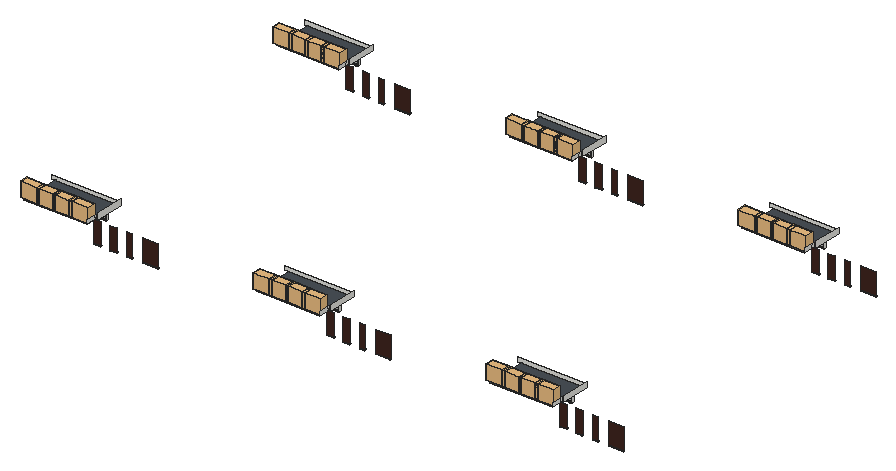
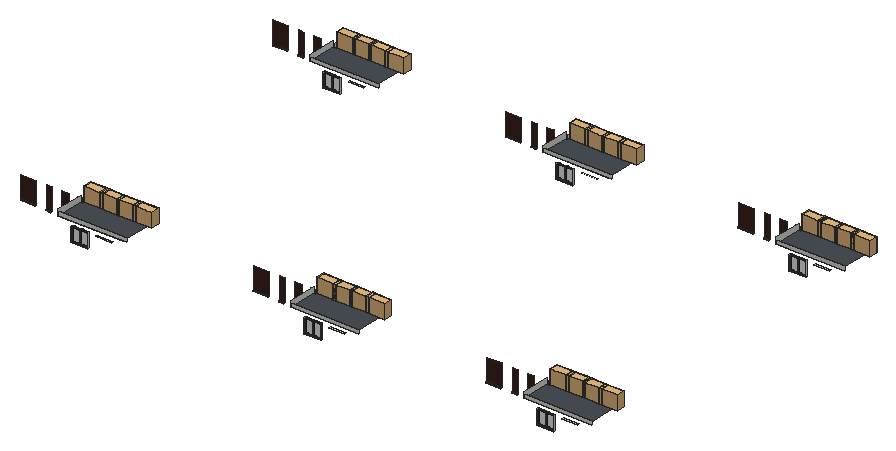
# SketchUp Ruby script. Lengths in inches.
U = 1.inch
M = Sketchup.active_model
def pt(a) = Geom::Point3d.new(a.map { |v| v * U })
def face(e, loops, mat)
  f = e.add_face(loops[0].map { |a| pt(a) })
  loops[1..].each { |l| e.add_face(l.map { |a| pt(a) }).erase! }
  f.material = f.back_material = mat if mat
  f
end
# faces: each face lists its corners as indices into pts; further lists are holes
def faces(e, pts, list, mat = nil) = list.each { |f| face(e, (f[0].is_a?(Array) ? f : [f]).map { |l| l.map { |i| pts[i] } }, mat) }
# xy, xz, yz: faces in a plane at the given z, y or x. An outline is a flat list of corners, or four numbers for a rectangle; further outlines are holes
def ring(l) = l.size == 4 ? [[l[0], l[1]], [l[2], l[1]], [l[2], l[3]], [l[0], l[3]]] : l.each_slice(2).to_a
def flat(e, list, mat, &to3) = list.each { |f| face(e, (f[0].is_a?(Array) ? f : [f]).map { |l| ring(l).map { |u, v| to3.(u, v) } }, mat) }
def xy(e, z, list, mat = nil) = flat(e, list, mat) { |x, y| [x, y, z] }
def xz(e, y, list, mat = nil) = flat(e, list, mat) { |x, z| [x, y, z] }
def yz(e, x, list, mat = nil) = flat(e, list, mat) { |y, z| [x, y, z] }
def lines(e, pts, list) = list.each { |a, b| e.add_line(pt(pts[a]), pt(pts[b])) }
# prism: a flat outline (further loops are holes) pulled along v
def prism(e, loops, v, mat = nil)
  f = face(e, loops, mat); d = Geom::Vector3d.new(v.map { |x| x * U })
  f.pushpull(f.normal.samedirection?(d) ? d.length : -d.length)
end
def box(e, o, s, mat = nil) = prism(e, [[o, [o[0] + s[0], o[1], o[2]], [o[0] + s[0], o[1] + s[1], o[2]], [o[0], o[1] + s[1], o[2]]]], [0, 0, s[2]], mat)
def at(x, y, z, deg = 0) = Geom::Transformation.translation(pt([x, y, z])) * Geom::Transformation.rotation(ORIGIN, Z_AXIS, deg.degrees)
def axes(o, x, y, z) = Geom::Transformation.new([*x, 0, *y, 0, *z, 0, *pt(o).to_a, 1])
def part(name) = M.definitions.add(name)
# library, detail: a bought-in or finely detailed component or shape, given as its bounding box
def library(name, o, s) = part(name).tap { |d| box(d.entities, o, s) }
def detail(e, o, s) = box(e.add_group.entities, o, s)
def put(e, d, t, mat = nil) = e.add_instance(d, t).tap { |i| i.material = mat if mat }
def group(e, t, mat = nil) = e.add_group.tap { |g| g.transformation = t; g.material = mat if mat }.entities
root = M.entities
M.materials.add("Glass_Tinted_Gray").color = [0, 0, 0]
M.materials["Glass_Tinted_Gray"].alpha = 0.125
M.materials.add("[0043_SaddleBrown]").color = [63, 38, 31]
M.materials.add("[0135_DarkGray]").color = [81, 81, 81]
M.materials.add("[Formica Blue]").color = [73, 80, 86]
M.materials.add("[Mirror 02]").color = [229, 229, 229]
M.materials.add("[Terrazzo Light Blue]").color = [196, 214, 227]
c1 = part("PENTEK_RP Fineline 50S_Sliding_DoorCase_E1")
box(c1.entities,[0,0,0],[1.51,3.66,99.27],"[0135_DarkGray]")
c2 = part("PENTEK_RP Fineline 50S_SlidingDooe_Case_E2")
box(c2.entities,[0,0,0],[96.25,3.66,1.51],"[0135_DarkGray]")
c3 = part("pentek_RP Fineline 50S_SlidingDoor_Case")
put(c3.entities,c1,at(97.76,0,0))
put(c3.entities,c2,at(1.51,0,0))
put(c3.entities,c1,at(0,0,0))
put(c3.entities,c2,at(1.51,0,97.76))
c4 = part("PENTEK_RP Fineline 50S_SlidingDoor_GlazingBead_2")
box(c4.entities,[0,0,0],[0.56,0.59,94.39],"[0135_DarkGray]")
c5 = part("PENTEK_RP Fineline 50S_SlidingDoor_Glass")
box(c5.entities,[0,0,0],[46.58,0.16,94.39],"Glass_Tinted_Gray")
c6 = part("PENTEK_RP Fineline 50S_SlidingDoor_GlazingBead")
box(c6.entities,[0,0,0],[45.47,0.59,0.56],"[0135_DarkGray]")
c7 = part("PENTEK_RP Fineline 50S_SlidingDoor_Leaf_E1")
xy(c7.entities,0,[[0,0,0.93,1.97],[0.93,1.57,1.49,1.97]],"[0135_DarkGray]")
xy(c7.entities,96.25,[[0,0,0.93,0,0.93,1.57,1.49,1.57,1.49,1.97,0,1.97]],"[0135_DarkGray]")
xz(c7.entities,0,[[0,0,0.93,96.25]],"[0135_DarkGray]")
xz(c7.entities,1.57,[[0.93,0,1.49,95.32],[0.93,95.32,1.49,96.25]],"[0135_DarkGray]")
xz(c7.entities,1.97,[[0,0,1.49,96.25]],"[0135_DarkGray]")
yz(c7.entities,0,[[0,0,1.97,96.25]],"[0135_DarkGray]")
yz(c7.entities,0.93,[[0,0,1.57,0.93],[0,0.93,1.57,95.32],[0,95.32,1.57,96.25]],"[0135_DarkGray]")
yz(c7.entities,1.49,[[1.57,0,1.97,95.32],[1.57,95.32,1.97,96.25]],"[0135_DarkGray]")
c8 = part("PENTEK_RP Fineline 50S_SlidingDoor_Leaf_E2")
xy(c8.entities,0,[[0,0,0,1.57,0.56,1.57,0.56,1.97,46.02,1.97,46.02,1.57,46.58,1.57,46.58,0]],"[0135_DarkGray]")
xy(c8.entities,0.93,[[0,0,46.58,1.57]],"[0135_DarkGray]")
xy(c8.entities,1.49,[[0.56,1.57,46.02,1.97]],"[0135_DarkGray]")
xz(c8.entities,0,[[0,0,46.58,0.93]],"[0135_DarkGray]")
xz(c8.entities,1.57,[[0,0,0.56,0.93],[46.02,0,46.58,0.93],[0.56,0.93,46.02,1.49]],"[0135_DarkGray]")
xz(c8.entities,1.97,[[0.56,0,46.02,1.49]],"[0135_DarkGray]")
yz(c8.entities,0,[[0,0,1.57,0.93]],"[0135_DarkGray]")
yz(c8.entities,0.56,[[1.57,0,1.97,0.93],[1.57,0.93,1.97,1.49]],"[0135_DarkGray]")
yz(c8.entities,46.02,[[1.57,0,1.97,0.93],[1.57,0.93,1.97,1.49]],"[0135_DarkGray]")
yz(c8.entities,46.58,[[0,0,1.57,0.93]],"[0135_DarkGray]")
c9 = part("PENTEK_RP Fineline S_SlidingDoor_Leaf1")
put(c9.entities,c4,at(0.93,0,0.93))
put(c9.entities,c4,at(46.96,0,0.93))
put(c9.entities,c5,at(1.49,1.42,0.93))
put(c9.entities,c6,at(1.49,0,0.93))
put(c9.entities,c5,at(1.49,0.59,0.93),"[Terrazzo Light Blue]")
put(c9.entities,c7,at(0,0,0))
put(c9.entities,c7,axes([48.44,0,0],[-1,0,0],[0,1,0],[0,0,1]))
put(c9.entities,c8,axes([0.93,0,96.25],[1,0,0],[0,1,0],[0,0,-1]))
put(c9.entities,c8,at(0.93,0,0))
put(c9.entities,c6,at(1.49,0,94.77))
c10 = part("PENTEK_RP Fineline 50S_SlidingDoor_Leaf2")
put(c10.entities,c5,at(1.49,1.42,0.93))
put(c10.entities,c6,at(1.49,0,94.77))
put(c10.entities,c4,at(46.96,0,0.93))
put(c10.entities,c5,at(1.49,0.59,0.93),"[Mirror 02]")
put(c10.entities,c4,at(0.93,0,0.93))
put(c10.entities,c7,at(0,0,0))
put(c10.entities,c7,axes([48.44,0,0],[-1,0,0],[0,1,0],[0,0,1]))
put(c10.entities,c6,at(1.49,0,0.93))
put(c10.entities,c8,axes([0.93,0,96.25],[1,0,0],[0,1,0],[0,0,-1]))
put(c10.entities,c8,at(0.93,0,0))
c11 = part("PENTEK - Slimmest Steel Sliding Door / Window\#1")
put(c11.entities,c3,at(0,-1.88,-0.09))
put(c11.entities,c9,at(1.51,-2.27,1.42))
put(c11.entities,c10,at(49.32,-0.3,1.42))
c12 = library("Group13",[-203.48,36.63,0],[29.68,67.31,50.64])
xy(root,173.82,[[451.01,438.72,467.3,441.04],[1175.45,438.72,1191.74,441.04],[1899.89,438.72,1916.17,441.04],[451.01,1419.07,467.3,1421.39],[1175.45,1419.07,1191.74,1421.39],
  [1899.89,1419.07,1916.17,1421.39]])
xy(root,173.87,[[419.76,438.72,419.76,441.04,399.16,441.04,399.16,438.73],[1144.2,438.72,1144.2,441.04,1123.6,441.04,1123.6,438.73],[1868.64,438.72,1868.64,441.04,1848.04,441.04,1848.04,438.73],[419.76,1419.07,419.76,1421.39,399.16,1421.39,399.16,1419.08],[1144.2,1419.07,1144.2,1421.39,1123.6,1421.39,1123.6,1419.08],
  [1868.64,1419.07,1868.64,1421.39,1848.04,1421.39,1848.04,1419.08]])
xy(root,174.69,[[348.1875,438.72,370.54,441.04],[1072.625,438.72,1094.98,441.04],[1797.0625,438.72,1819.41,441.04],[348.1875,1419.07,370.54,1419.08,370.54,1421.39,348.1875,1421.39],[1072.625,1419.07,1094.98,1419.08,1094.98,1421.39,1072.625,1421.39],
  [1797.0625,1419.07,1819.41,1419.08,1819.41,1421.39,1797.0625,1421.39]])
xy(root,174.81,[[500.42,438.73,547.05,441.04],[1224.86,438.73,1271.49,441.04],[1949.3,438.73,1995.93,441.04],[500.42,1419.08,547.05,1421.39],[1224.86,1419.08,1271.49,1421.39],
  [1949.3,1419.08,1995.93,1421.39]])
xy(root,175.12,[[419.76,438.72,399.16,438.73,399.16,441.04,419.76,441.04],[1144.2,438.72,1123.6,438.73,1123.6,441.04,1144.2,441.04],[1868.64,438.72,1848.04,438.73,1848.04,441.04,1868.64,441.04],[419.76,1419.07,399.16,1419.08,399.16,1421.39,419.76,1421.39],[1144.2,1419.07,1123.6,1419.08,1123.6,1421.39,1144.2,1421.39],
  [1868.64,1419.07,1848.04,1419.08,1848.04,1421.39,1868.64,1421.39]])
xy(root,175.93,[[451.01,438.72,467.3,441.04],[1175.45,438.72,1191.74,441.04],[1899.89,438.72,1916.17,441.04],[451.01,1419.07,467.3,1421.39],[1175.45,1419.07,1191.74,1421.39],
  [1899.89,1419.07,1916.17,1421.39]])
xy(root,176.39,[[348.1875,438.72,370.54,441.04],[1072.625,438.72,1094.98,441.04],[1797.0625,438.72,1819.41,441.04],[348.1875,1419.07,370.54,1421.39],[1072.625,1419.07,1094.98,1421.39],
  [1797.0625,1419.07,1819.41,1421.39]])
xy(root,177.22,[[500.42,438.73,547.05,441.04],[1224.86,438.73,1271.49,441.04],[1949.3,438.73,1995.93,441.04],[500.42,1419.08,547.05,1421.39],[1224.86,1419.08,1271.49,1421.39],
  [1949.3,1419.08,1995.93,1421.39]])
xy(root,183.6875,[[258.09,535.375,309.84,540.48],[982.53,535.375,1034.28,540.48],[1706.96,535.375,1758.71,540.48],[258.09,1515.73,309.84,1520.83],[982.53,1515.73,1034.28,1520.83],
  [1706.96,1515.73,1758.71,1520.83]])
xy(root,227.875,[[183.3,535.375,231.3,540.48],[258.09,535.375,309.84,540.48],[907.74,535.375,955.74,540.48],[982.53,535.375,1034.28,540.48],[1632.17,535.375,1680.17,540.48],
  [1706.96,535.375,1758.71,540.48],[183.3,1515.73,231.3,1520.83],[258.09,1515.73,309.84,1520.83],[907.74,1515.73,955.74,1520.83],[982.53,1515.73,1034.28,1520.83],
  [1632.17,1515.73,1680.17,1520.83],[1706.96,1515.73,1758.71,1520.83]])
xy(root,240.625,[[[153.26,412.04,153.26,535.375,353.97,535.375,353.97,447.84,348.1875,447.84,348.1875,412.04],[154.69,414.01,158.32,418.7],[160.01,414.01,163.63,418.7],[165.19,414.01,168.82,418.7],[170.38,414.01,174.01,418.7],[181.38,414.01,185.01,418.7],[186.88,414.01,190.51,418.7],[192.38,414.01,196.01,418.7],[197.88,414.01,201.51,418.7],[203.38,414.01,207.01,418.7],[175.88,414.01,179.51,418.7]],[[877.69,412.04,877.69,535.375,1078.41,535.375,1078.41,447.84,1072.625,447.84,1072.625,412.04],[879.13,414.01,882.76,418.7],[884.44,414.01,888.07,418.7],[889.63,414.01,893.26,418.7],[894.82,414.01,898.44,418.7],[900.32,414.01,903.94,418.7],[905.82,414.01,909.44,418.7],[911.32,414.01,914.94,418.7],[916.82,414.01,920.44,418.7],[922.32,414.01,925.94,418.7],[927.82,414.01,931.44,418.7]],[[1602.13,412.04,1602.13,535.375,1802.84,535.375,1802.84,447.84,1797.0625,447.84,1797.0625,412.04],[1603.57,414.01,1607.19,418.7],[1608.88,414.01,1612.51,418.7],[1614.07,414.01,1617.69,418.7],[1619.26,414.01,1622.88,418.7],[1630.26,414.01,1633.88,418.7],[1635.76,414.01,1639.38,418.7],[1641.26,414.01,1644.88,418.7],[1646.76,414.01,1650.38,418.7],[1652.26,414.01,1655.88,418.7],[1624.76,414.01,1628.38,418.7]],[[153.26,1392.39,153.26,1515.73,353.97,1515.73,353.97,1428.19,348.1875,1428.19,348.1875,1392.39],[154.69,1394.36,158.32,1399.05],[160.01,1394.36,163.63,1399.05],[165.19,1394.36,168.82,1399.05],[170.38,1394.36,174.01,1399.05],[181.38,1394.36,185.01,1399.05],[186.88,1394.36,190.51,1399.05],[192.38,1394.36,196.01,1399.05],[197.88,1394.36,201.51,1399.05],[203.38,1394.36,207.01,1399.05],[175.88,1394.36,179.51,1399.05]],[[877.69,1392.39,877.69,1515.73,1078.41,1515.73,1078.41,1428.19,1072.625,1428.19,1072.625,1392.39],[879.13,1394.36,882.76,1399.05],[884.44,1394.36,888.07,1399.05],[889.63,1394.36,893.26,1399.05],[894.82,1394.36,898.44,1399.05],[900.32,1394.36,903.94,1399.05],[905.82,1394.36,909.44,1399.05],[911.32,1394.36,914.94,1399.05],[916.82,1394.36,920.44,1399.05],[922.32,1394.36,925.94,1399.05],[927.82,1394.36,931.44,1399.05]],
  [[1602.13,1392.39,1602.13,1515.73,1802.84,1515.73,1802.84,1428.19,1797.0625,1428.19,1797.0625,1392.39],[1603.57,1394.36,1607.19,1399.05],[1608.88,1394.36,1612.51,1399.05],[1614.07,1394.36,1617.69,1399.05],[1619.26,1394.36,1622.88,1399.05],[1630.26,1394.36,1633.88,1399.05],[1635.76,1394.36,1639.38,1399.05],[1641.26,1394.36,1644.88,1399.05],[1646.76,1394.36,1650.38,1399.05],[1652.26,1394.36,1655.88,1399.05],[1624.76,1394.36,1628.38,1399.05]]],"[Formica Blue]")
xz(root,438.72,[[451.01,175.93,467.3,243.96],[1175.45,175.93,1191.74,243.96],[1899.89,175.93,1916.17,243.96],[348.1875,176.39,370.54,243.96],[1072.625,176.39,1094.98,243.96],
  [1797.0625,176.39,1819.41,243.96]],"[0043_SaddleBrown]")
xz(root,438.73,[[500.42,177.22,547.05,243.96],[1224.86,177.22,1271.49,243.96],[1949.3,177.22,1995.93,243.96]],"[0043_SaddleBrown]")
xz(root,441.04,[[451.01,173.82,467.3,175.93],[1175.45,173.82,1191.74,175.93],[1899.89,173.82,1916.17,175.93],[399.16,173.87,419.76,175.12],[1123.6,173.87,1144.2,175.12],
  [1848.04,173.87,1868.64,175.12],[348.1875,174.69,370.54,176.39],[1072.625,174.69,1094.98,176.39],[1797.0625,174.69,1819.41,176.39],[500.42,174.81,547.05,177.22],
  [1224.86,174.81,1271.49,177.22],[1949.3,174.81,1995.93,177.22]],"[0043_SaddleBrown]")
xz(root,447.84,[[348.1875,240.625,353.97,252.25],[1072.625,240.625,1078.41,252.25],[1797.0625,240.625,1802.84,252.25]])
xz(root,535.375,[[141.63,240.625,353.97,252.25],[866.07,240.625,1078.41,252.25],[1590.51,240.625,1802.84,252.25]])
xz(root,1419.07,[[451.01,175.93,467.3,243.96],[1175.45,175.93,1191.74,243.96],[1899.89,175.93,1916.17,243.96],[348.1875,176.39,370.54,243.96],[1072.625,176.39,1094.98,243.96],
  [1797.0625,176.39,1819.41,243.96]],"[0043_SaddleBrown]")
xz(root,1419.08,[[500.42,177.22,547.05,243.96],[1224.86,177.22,1271.49,243.96],[1949.3,177.22,1995.93,243.96]],"[0043_SaddleBrown]")
xz(root,1421.39,[[451.01,173.82,467.3,175.93],[1175.45,173.82,1191.74,175.93],[1899.89,173.82,1916.17,175.93],[399.16,173.87,419.76,175.12],[1123.6,173.87,1144.2,175.12],
  [1848.04,173.87,1868.64,175.12],[348.1875,174.69,370.54,176.39],[1072.625,174.69,1094.98,176.39],[1797.0625,174.69,1819.41,176.39],[500.42,174.81,547.05,177.22],
  [1224.86,174.81,1271.49,177.22],[1949.3,174.81,1995.93,177.22]],"[0043_SaddleBrown]")
xz(root,1428.19,[[348.1875,240.625,353.97,252.25],[1072.625,240.625,1078.41,252.25],[1797.0625,240.625,1802.84,252.25]])
xz(root,1515.73,[[141.63,240.625,353.97,252.25],[866.07,240.625,1078.41,252.25],[1590.51,240.625,1802.84,252.25]])
yz(root,258.09,[[535.375,183.6875,540.48,227.875],[1515.73,183.6875,1520.83,227.875]])
yz(root,309.84,[[535.375,183.6875,540.48,227.875],[1515.73,183.6875,1520.83,227.875]])
yz(root,348.1875,[[412.04,240.625,438.72,240.625,438.72,243.96,441.04,243.96,441.04,246.4375,438.72,246.4375,438.72,252.25,412.04,252.25],[438.72,240.625,438.72,243.96,441.04,243.96,441.04,246.4375,438.72,246.4375,438.72,252.25,447.84,252.25,447.84,240.625],[1392.39,240.625,1419.07,240.625,1419.07,243.96,1421.39,243.96,1421.39,246.4375,1419.07,246.4375,1419.07,252.25,1392.39,252.25],[1419.07,240.625,1419.07,243.96,1421.39,243.96,1421.39,246.4375,1419.07,246.4375,1419.07,252.25,1428.19,252.25,1428.19,240.625]])
yz(root,353.97,[[447.84,240.625,535.375,258.25],[1428.19,240.625,1515.73,258.25]])
yz(root,982.53,[[535.375,183.6875,540.48,227.875],[1515.73,183.6875,1520.83,227.875]])
yz(root,1034.28,[[535.375,183.6875,540.48,227.875],[1515.73,183.6875,1520.83,227.875]])
yz(root,1072.625,[[412.04,240.625,438.72,240.625,438.72,243.96,441.04,243.96,441.04,246.4375,438.72,246.4375,438.72,252.25,412.04,252.25],[438.72,240.625,438.72,243.96,441.04,243.96,441.04,246.4375,438.72,246.4375,438.72,252.25,447.84,252.25,447.84,240.625],[1392.39,240.625,1419.07,240.625,1419.07,243.96,1421.39,243.96,1421.39,246.4375,1419.07,246.4375,1419.07,252.25,1392.39,252.25],[1419.07,240.625,1419.07,243.96,1421.39,243.96,1421.39,246.4375,1419.07,246.4375,1419.07,252.25,1428.19,252.25,1428.19,240.625]])
yz(root,1078.41,[[447.84,240.625,535.375,258.25],[1428.19,240.625,1515.73,258.25]])
yz(root,1706.96,[[535.375,183.6875,540.48,227.875],[1515.73,183.6875,1520.83,227.875]])
yz(root,1758.71,[[535.375,183.6875,540.48,227.875],[1515.73,183.6875,1520.83,227.875]])
yz(root,1797.0625,[[412.04,240.625,438.72,240.625,438.72,243.96,441.04,243.96,441.04,246.4375,438.72,246.4375,438.72,252.25,412.04,252.25],[438.72,240.625,438.72,243.96,441.04,243.96,441.04,246.4375,438.72,246.4375,438.72,252.25,447.84,252.25,447.84,240.625],[1392.39,240.625,1419.07,240.625,1419.07,243.96,1421.39,243.96,1421.39,246.4375,1419.07,246.4375,1419.07,252.25,1392.39,252.25],[1419.07,240.625,1419.07,243.96,1421.39,243.96,1421.39,246.4375,1419.07,246.4375,1419.07,252.25,1428.19,252.25,1428.19,240.625]])
yz(root,1802.84,[[447.84,240.625,535.375,258.25],[1428.19,240.625,1515.73,258.25]])
p = [[399.16,438.72,243.96],[399.16,438.73,175.12],[419.76,438.72,175.12],[419.76,438.72,243.96],[1123.6,438.72,243.96],[1123.6,438.73,175.12],
  [1144.2,438.72,175.12],[1144.2,438.72,243.96],[1848.04,438.72,243.96],[1848.04,438.73,175.12],[1868.64,438.72,175.12],[1868.64,438.72,243.96],
  [399.16,1419.07,243.96],[399.16,1419.08,175.12],[419.76,1419.07,175.12],[419.76,1419.07,243.96],[1123.6,1419.07,243.96],[1123.6,1419.08,175.12],
  [1144.2,1419.07,175.12],[1144.2,1419.07,243.96],[1848.04,1419.07,243.96],[1848.04,1419.08,175.12],[1868.64,1419.07,175.12],[1868.64,1419.07,243.96]]
faces(root,p,[[0,1,2,3],[4,5,6,7],[8,9,10,11],[12,13,14,15],[16,17,18,19],[20,21,22,23]],"[0043_SaddleBrown]")
put(root,c11,axes([982.53,1516.55,183.73],[0.52129,0,0],[0,0.44,0],[0,0,0.44603]))
put(root,c11,axes([258.09,1516.55,183.73],[0.52129,0,0],[0,0.44,0],[0,0,0.44603]))
put(root,c11,axes([1706.96,1516.55,183.73],[0.52129,0,0],[0,0.44,0],[0,0,0.44603]))
put(root,c11,axes([982.53,536.2,183.73],[0.52129,0,0],[0,0.44,0],[0,0,0.44603]))
put(root,c11,axes([1706.96,536.2,183.73],[0.52129,0,0],[0,0.44,0],[0,0,0.44603]))
put(root,c11,axes([258.09,536.2,183.73],[0.52129,0,0],[0,0.44,0],[0,0,0.44603]))
put(root,c12,axes([829.65,1245.5,240.42],[0,-0.8723,0],[0.8723,0,0],[0,0,0.8723]))
put(root,c12,axes([930.96,1245.5,240.42],[0,-0.8723,0],[0.8723,0,0],[0,0,0.8723]))
put(root,c12,axes([879.59,1245.5,240.42],[0,-0.8723,0],[0.8723,0,0],[0,0,0.8723]))
put(root,c12,axes([980.65,1245.5,240.42],[0,-0.8723,0],[0.8723,0,0],[0,0,0.8723]))
put(root,c12,axes([1554.09,1245.5,240.42],[0,-0.8723,0],[0.8723,0,0],[0,0,0.8723]))
put(root,c12,axes([256.21,1245.5,240.42],[0,-0.8723,0],[0.8723,0,0],[0,0,0.8723]))
put(root,c12,axes([105.21,1245.5,240.42],[0,-0.8723,0],[0.8723,0,0],[0,0,0.8723]))
put(root,c12,axes([1705.09,1245.5,240.42],[0,-0.8723,0],[0.8723,0,0],[0,0,0.8723]))
put(root,c12,axes([206.53,1245.5,240.42],[0,-0.8723,0],[0.8723,0,0],[0,0,0.8723]))
put(root,c12,axes([155.15,1245.5,240.42],[0,-0.8723,0],[0.8723,0,0],[0,0,0.8723]))
put(root,c12,axes([1655.4,1245.5,240.42],[0,-0.8723,0],[0.8723,0,0],[0,0,0.8723]))
put(root,c12,axes([1604.03,1245.5,240.42],[0,-0.8723,0],[0.8723,0,0],[0,0,0.8723]))
put(root,c12,axes([829.65,265.15,240.42],[0,-0.8723,0],[0.8723,0,0],[0,0,0.8723]))
put(root,c12,axes([879.59,265.15,240.42],[0,-0.8723,0],[0.8723,0,0],[0,0,0.8723]))
put(root,c12,axes([930.96,265.15,240.42],[0,-0.8723,0],[0.8723,0,0],[0,0,0.8723]))
put(root,c12,axes([980.65,265.15,240.42],[0,-0.8723,0],[0.8723,0,0],[0,0,0.8723]))
put(root,c12,axes([1554.09,265.15,240.42],[0,-0.8723,0],[0.8723,0,0],[0,0,0.8723]))
put(root,c12,axes([1604.03,265.15,240.42],[0,-0.8723,0],[0.8723,0,0],[0,0,0.8723]))
put(root,c12,axes([1655.4,265.15,240.42],[0,-0.8723,0],[0.8723,0,0],[0,0,0.8723]))
put(root,c12,axes([1705.09,265.15,240.42],[0,-0.8723,0],[0.8723,0,0],[0,0,0.8723]))
put(root,c12,axes([105.21,265.15,240.42],[0,-0.8723,0],[0.8723,0,0],[0,0,0.8723]))
put(root,c12,axes([256.21,265.15,240.42],[0,-0.8723,0],[0.8723,0,0],[0,0,0.8723]))
put(root,c12,axes([206.53,265.15,240.42],[0,-0.8723,0],[0.8723,0,0],[0,0,0.8723]))
put(root,c12,axes([155.15,265.15,240.42],[0,-0.8723,0],[0.8723,0,0],[0,0,0.8723]))
